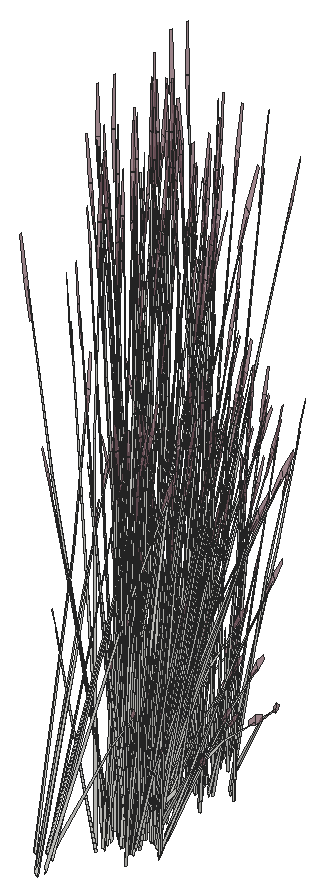
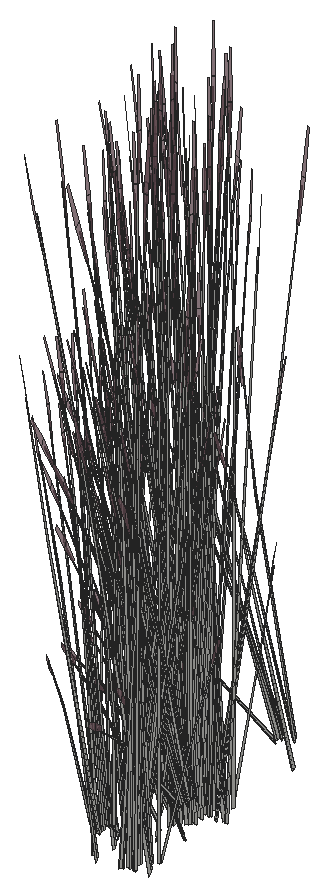
# SketchUp Ruby script. Lengths in inches.
U = 1.inch
M = Sketchup.active_model
def pt(a) = Geom::Point3d.new(a.map { |v| v * U })
def face(e, loops, mat)
  f = e.add_face(loops[0].map { |a| pt(a) })
  loops[1..].each { |l| e.add_face(l.map { |a| pt(a) }).erase! }
  f.material = f.back_material = mat if mat
  f
end
# faces: each face lists its corners as indices into pts; further lists are holes
def faces(e, pts, list, mat = nil) = list.each { |f| face(e, (f[0].is_a?(Array) ? f : [f]).map { |l| l.map { |i| pts[i] } }, mat) }
# xy, xz, yz: faces in a plane at the given z, y or x. An outline is a flat list of corners, or four numbers for a rectangle; further outlines are holes
def ring(l) = l.size == 4 ? [[l[0], l[1]], [l[2], l[1]], [l[2], l[3]], [l[0], l[3]]] : l.each_slice(2).to_a
def flat(e, list, mat, &to3) = list.each { |f| face(e, (f[0].is_a?(Array) ? f : [f]).map { |l| ring(l).map { |u, v| to3.(u, v) } }, mat) }
def xy(e, z, list, mat = nil) = flat(e, list, mat) { |x, y| [x, y, z] }
def xz(e, y, list, mat = nil) = flat(e, list, mat) { |x, z| [x, y, z] }
def yz(e, x, list, mat = nil) = flat(e, list, mat) { |y, z| [x, y, z] }
def lines(e, pts, list) = list.each { |a, b| e.add_line(pt(pts[a]), pt(pts[b])) }
# prism: a flat outline (further loops are holes) pulled along v
def prism(e, loops, v, mat = nil)
  f = face(e, loops, mat); d = Geom::Vector3d.new(v.map { |x| x * U })
  f.pushpull(f.normal.samedirection?(d) ? d.length : -d.length)
end
def box(e, o, s, mat = nil) = prism(e, [[o, [o[0] + s[0], o[1], o[2]], [o[0] + s[0], o[1] + s[1], o[2]], [o[0], o[1] + s[1], o[2]]]], [0, 0, s[2]], mat)
def at(x, y, z, deg = 0) = Geom::Transformation.translation(pt([x, y, z])) * Geom::Transformation.rotation(ORIGIN, Z_AXIS, deg.degrees)
def axes(o, x, y, z) = Geom::Transformation.new([*x, 0, *y, 0, *z, 0, *pt(o).to_a, 1])
def part(name) = M.definitions.add(name)
# library, detail: a bought-in or finely detailed component or shape, given as its bounding box
def library(name, o, s) = part(name).tap { |d| box(d.entities, o, s) }
def detail(e, o, s) = box(e.add_group.entities, o, s)
def put(e, d, t, mat = nil) = e.add_instance(d, t).tap { |i| i.material = mat if mat }
def group(e, t, mat = nil) = e.add_group.tap { |g| g.transformation = t; g.material = mat if mat }.entities
root = M.entities
M.materials.add("LightPink_Translucent").color = [144, 107, 117]
M.materials["LightPink_Translucent"].alpha = 0.75
c1 = part("blade")
p = [[2.15,0.21,22],[0,0.17,0],[0.09,0.45,0],[2.18,0.31,22],[2.29,0.31,22],[0.38,0.45,0],
  [2.48,0.24,33],[2.49,0.24,33],[2.48,0.22,33]]
faces(c1.entities,p,[[0,1,2,3],[4,5,2,3],[6,3,4,7],[8,0,3,6]])
c2 = part("seeds")
p = [[0.3,-0.1,1.38],[-0.01,-0.03,1.59],[-0.01,-0.03,0.03],[0.14,-0.07,-0.07],[0.29,-0.03,3],[0.15,0.01,3.11]]
faces(c2.entities,p,[[0,1,2,3],[1,0,4,5]],"LightPink_Translucent")
c3 = part("blade with seeds")
put(c3.entities,c1,at(0,0,0))
put(c3.entities,c2,axes([2.4,0.25,30.99],[1.5799,-0.05474,1.17369],[-0.12525,1.92788,0.29478],[-0.07173,-0.02425,1.56792]))
put(root,c3,axes([406.99,322.08,-7.34],[0.3661,0.36521,-0.52818],[-0.38674,0.31985,-0.40911],[-0.0557,0.18556,1.01061]))
put(root,c3,axes([406.6,322.63,-9.37],[0.46459,-0.09625,0.0606],[0.10681,0.38778,-0.80367],[-0.02945,0.1963,0.72038]))
put(root,c3,axes([408.08,322.43,-7.64],[0.50273,0.13626,-0.47583],[-0.17232,0.46717,-0.36857],[0.0461,0.18809,0.91046]))
put(root,c3,axes([408.37,321.47,-8.39],[-0.1169,-0.17452,1.59586],[0.54019,-0.14692,0.12904],[0.12209,0.27397,0.68222]))
put(root,c3,axes([407.85,322.72,-7.78],[-0.15418,0.41799,-0.32977],[-0.44981,-0.12192,0.42575],[0.04124,0.16829,0.81462]))
put(root,c3,axes([406.84,330.74,-10.05],[-0.21003,-0.55738,-0.65031],[0.60499,-0.20074,-0.17068],[-0.02321,-0.18874,1.43544]))
put(root,c3,axes([409.65,329.04,-10.61],[-0.07655,-0.04282,1.6421],[-0.19662,-0.47839,-0.25086],[0.13264,-0.12982,0.2797]))
put(root,c3,axes([407.41,321.56,-8.39],[-0.01252,-0.20862,1.59586],[0.54251,0.1384,0.12904],[-0.03356,0.2973,0.68222]))
put(root,c3,axes([408.07,329.15,-7.3],[-0.15418,0.41799,0.32977],[-0.44981,-0.12192,-0.42575],[-0.04124,-0.16829,0.81462]))
put(root,c3,axes([409.22,329.32,-7.59],[0.36417,0.37086,0.447],[-0.38674,0.31985,0.36857],[0.06718,-0.174,0.92496]))
put(root,c3,axes([409.35,329.36,-7.6],[0.42027,0.02533,0.05988],[-0.01152,0.38243,0.47138],[0.04398,-0.14649,0.71878]))
put(root,c3,axes([407.9,322.35,-7.36],[0.24409,0.44196,-0.66157],[-0.50245,0.2463,0.07984],[0.05708,0.21354,0.93586]))
put(root,c3,axes([409.04,329.62,-7.3],[-0.34603,0.28618,0.32977],[-0.32756,-0.32677,-0.42575],[0.04984,-0.16603,0.81462]))
put(root,c3,axes([409.65,330.39,-7.36],[0.26714,-0.42887,-0.66157],[0.46811,0.30479,0.07984],[0.1595,-0.15539,0.93586]))
put(root,c3,axes([406.76,329.14,-9.79],[-0.31974,-0.54466,0],[0.53494,-0.30375,-0.48057],[0.12184,-0.06918,1.52448]))
put(root,c3,axes([409.64,330.1875,-7.64],[-0.13138,-0.49631,-0.47583],[0.49754,-0.08682,-0.36857],[0.14258,-0.13331,0.91046]))
put(root,c3,axes([407.53,323.46,-7.61],[0.06483,0.08753,1.62908],[0.52315,0.03439,-0.25764],[0.05261,0.19303,0.13065]))
put(root,c3,axes([407.46,328.48,-10.02],[-0.35341,0.31182,-0.03625],[-0.32382,-0.34152,-0.16435],[-0.0228,-0.09677,0.54209]))
put(root,c3,axes([409.87,330.54,-7.3125],[-0.47307,-0.29971,-0.11324],[0.27254,-0.43404,-0.62851],[0.13365,-0.15087,0.95501]))
put(root,c3,axes([407.2,329.05,-10.12],[0.47863,-0.27177,-0.46235],[0.28609,0.48733,0],[0.10901,-0.0619,1.46668]))
put(root,c3,axes([410.04,329.99,-9.59],[-0.1827,-0.0161,1.33163],[-0.18717,-0.43188,-0.28638],[0.22444,-0.12218,0.56934]))
put(root,c3,axes([411.04,330.41,-7.62],[-0.0668,-0.00413,1.65179],[-0.27738,-0.44233,-0.15608],[0.11139,-0.14544,0.29231]))
put(root,c3,axes([407.76,330.17,-10.08],[0.34446,-0.40855,-0.58063],[0.42791,0.37046,-0.15239],[0.13803,-0.10191,1.28164]))
put(root,c3,axes([410.25,329.2,-9.42],[-0.17034,0.27669,1.06958],[-0.14642,-0.37174,0.78586],[0.14069,-0.09315,0.23558]))
put(root,c3,axes([410,330.24,-7.78],[0.44516,-0.07768,-0.32977],[0.11755,0.44407,0.42575],[0.12757,-0.11927,0.81462]))
put(root,c3,axes([407.16,330.89,-9.94],[0.24813,-0.48978,-0.41661],[0.51557,0.23571,0.2005],[0,-0.1129,1.33761]))
put(root,c3,axes([407.39,330.64,-9.52],[-0.05959,-0.62022,-0.27094],[0.62068,-0.0375,-0.46562],[0.1093,-0.08261,1.4872]))
put(root,c3,axes([405.85,330.68,-10.11],[0.35699,-0.33913,-0.28847],[0.35699,0.33913,0.28847],[0,-0.10923,1.29413]))
put(root,c3,axes([409.64,330.5,-7.3],[-0.44516,0.07768,0.32977],[-0.11755,-0.44407,-0.42575],[0.12757,-0.11927,0.81462]))
put(root,c3,axes([407.31,329.27,-10.11],[0.47712,0.13449,-0.28847],[-0.12013,0.47362,0.28847],[0.09619,-0.05462,1.29413]))
put(root,c3,axes([410.04,330.43,-7.6],[0.35109,0.22859,0.05988],[-0.2044,0.32553,0.47138],[0.11256,-0.10524,0.71878]))
put(root,c3,axes([409.95,330.34,-7.59],[0.12683,0.50025,0.447],[-0.49754,0.08682,0.36857],[0.14663,-0.11765,0.92496]))
put(root,c3,axes([411.29,330.94,-7.61],[0.07097,-0.08279,1.62908],[-0.09083,-0.50786,-0.25764],[0.17806,-0.09629,0.13065]))
put(root,c3,axes([407.47,331.13,-9.73],[0.57623,0.26344,0.22409],[-0.27732,0.5474,0.46562],[0,-0.12618,1.49497]))
put(root,c3,axes([407.29,330.76,-9.47],[-0.55535,0.03355,0.41661],[-0.05022,-0.55698,-0.2005],[0.09942,-0.05645,1.33761]))
put(root,c3,axes([409.89,331.71,-7.3125],[-0.25732,-0.49218,-0.11324],[0.45669,-0.24187,-0.62851],[0.19245,-0.06494,0.95501]))
put(root,c3,axes([409.87,331.29,-7.64],[0.13855,-0.49442,-0.47583],[0.47502,0.16947,-0.36857],[0.19125,-0.04534,0.91046]))
put(root,c3,axes([409.12,329.28,-9.79],[0.31974,-0.54466,0],[0.53494,0.30375,-0.48057],[0.12184,0.06918,1.52448]))
put(root,c3,axes([407.27,330.96,-9.8],[0.22235,0.6078,0.42607],[-0.63531,0.21135,0.16719],[0.00776,-0.11168,1.47927]))
put(root,c3,axes([410.375,331.43,-10.15],[-0.32938,0.06523,1.31842],[-0.05243,-0.51922,0.07547],[0.2307,-0.07859,0.75023]))
put(root,c3,axes([410.98,330.97,-9.89],[-0.31706,-0.34757,-0.06041],[0.34725,-0.31847,-0.27392],[0.09839,-0.02242,0.90349]))
put(root,c3,axes([407.15,331.44,-9.47],[-0.24813,0.48978,0.41661],[-0.51557,-0.23571,-0.2005],[0,-0.1129,1.33761]))
put(root,c3,axes([408.07,331.01,-9.95],[0,-0.62892,0],[0.63949,0,0],[0,0,1.6711]))
put(root,c3,axes([408.84,329.5625,-9.69],[-0.47863,-0.27177,0.46235],[0.28609,-0.48733,0],[0.10901,0.0619,1.46668]))
put(root,c3,axes([409.78,331.47,-7.36],[0.44939,-0.24006,-0.66157],[0.25044,0.49415,0.07984],[0.21713,-0.05613,0.93586]))
put(root,c3,axes([407.76,330.62,-9.8],[-0.42403,0.49328,0.42607],[-0.50377,-0.43543,0.16719],[0.10223,-0.04923,1.47927]))
put(root,c3,axes([408.23,331.5,-9.86],[-0.47569,-0.46784,-0.05709],[0.47598,-0.46812,0],[-0.01661,-0.01634,1.63492]))
put(root,c3,axes([407.03,329.81,-9.7],[-0.14774,0.54019,0.16428],[-0.54062,-0.15287,0.32672],[0.09339,-0.00263,1.49371]))
put(root,c3,axes([409.71,331.5625,-7.3],[-0.42502,-0.15163,0.32977],[0.12396,-0.44238,-0.42575],[0.17112,-0.04056,0.81462]))
put(root,c3,axes([406.8,330.24,-10.52],[-0.50338,0.21762,1.20058],[-0.16022,-0.62439,0.4665],[0.30911,0.01039,1.36553]))
put(root,c3,axes([408.16,330.41,-9.5625],[0.09866,-0.48509,0.13483],[0.48202,0.0842,-0.38503],[0.08772,0.04981,1.18024]))
put(root,c3,axes([407.32,331.56,-9.8],[0.64638,0.11452,0.42607],[-0.13155,0.64678,0.16719],[-0.09446,-0.06245,1.47927]))
put(root,c3,axes([410.73,331.09,-10.61],[-0.02673,-0.08252,1.6421],[0.18538,-0.48271,-0.25086],[0.187,-0.00694,0.2797]))
put(root,c3,axes([407.95,330.53,-9.47],[-0.30722,-0.45622,0.41661],[0.46535,-0.32126,-0.2005],[0.09942,0.05645,1.33761]))
put(root,c3,axes([406.97,332.59,-9.7],[0.54955,-0.14427,0.16428],[0.1357,0.53689,0.32672],[-0.04901,-0.07823,1.49371]))
put(root,c3,axes([408.11,330.5625,-9.52],[0.51635,-0.36087,-0.27094],[0.34336,0.5099,-0.46562],[0.1274,0.05178,1.4872]))
put(root,c3,axes([410.16,331.51,-7.78],[0.42502,0.15163,-0.32977],[-0.12396,0.44238,0.42575],[0.17112,-0.04056,0.81462]))
put(root,c3,axes([409.41,329.6,-10.12],[0.47863,0.27177,-0.46235],[-0.28609,0.48733,0],[0.10901,0.0619,1.46668]))
put(root,c3,axes([408.5,331.15,-9.95],[0.57217,0,0],[0,0.56272,0],[0,0,1.66132]))
put(root,c3,axes([408.66,329.83,-9.7],[-0.54955,0.14427,0.16428],[-0.1357,-0.53689,0.32672],[0.04901,0.07823,1.49371]))
put(root,c3,axes([409,330.97,-8.39],[-0.21212,0.01231,1.59586],[0.14072,-0.53355,0.12904],[0.3023,0.033,0.68222]))
put(root,c3,axes([409.27,329.81,-10.11],[0.12013,0.47362,-0.28847],[-0.47712,0.13449,0.28847],[0.09619,0.05462,1.29413]))
put(root,c3,axes([410.1,331.7,-7.6],[0.18783,0.37061,0.05988],[-0.34252,0.1814,0.47138],[0.15099,-0.03579,0.71878]))
put(root,c3,axes([408.31,330.87,-9.78],[-0.64638,-0.11452,0.45814],[0.13155,-0.64678,0.17978],[0.09446,0.06245,1.59061]))
put(root,c3,axes([410.06,331.57,-7.59],[-0.14449,0.4956,0.447],[-0.47502,-0.16947,0.36857],[0.1868,-0.02978,0.92496]))
put(root,c3,axes([407.8,332.46,-9.95],[-0.16686,-0.46861,0],[0.47648,-0.16411,0],[0,0,1.4375]))
put(root,c3,axes([408.42,332.4,-9.97],[0.53691,-0.18442,-0.17877],[0.18866,0.53125,0.00007],[0.05927,-0.02038,1.61933]))
put(root,c3,axes([408.61,332.62,-9.7],[0.14774,-0.54019,0.16428],[0.54062,0.15287,0.32672],[-0.09339,0.00263,1.49371]))
put(root,c3,axes([408.49,331.4,-9.9375],[0.35699,0.35109,0],[-0.35699,0.35109,0],[0,0,1.57621]))
put(root,c3,axes([409.45,331.24,-9.7],[-0.40181,-0.39593,0.16428],[0.40492,-0.38402,0.32672],[-0.04438,0.08086,1.49371]))
put(root,c3,axes([408.71,330.64,-10.08],[0.53199,0.08911,-0.58063],[-0.11226,0.54969,-0.15239],[0.15876,0.06661,1.28164]))
put(root,c3,axes([411.0625,331.6,-9.42],[-0.31598,0.08973,1.06958],[0.14873,-0.37085,0.78586],[0.16763,0.02538,0.23558]))
put(root,c3,axes([407.68,332.68,-9.95],[-0.51557,-0.24403,0],[0.24813,-0.50705,0],[0,0,1.51513]))
put(root,c3,axes([408.48,330.98,-9.47],[0.24813,-0.48978,0.41661],[0.51557,0.23571,-0.2005],[0,0.1129,1.33761]))
put(root,c3,axes([410.91,333.17,-7.62],[-0.04624,-0.04758,1.65179],[0.10116,-0.51007,-0.15608],[0.18215,-0.03259,0.29231]))
put(root,c3,axes([408.39,331.27,-9.87],[0,0.62861,-0.05249],[-0.63949,0,0],[0,0.01975,1.67027]))
put(root,c3,axes([408.43,330.82,-9.94],[0.30722,0.45622,-0.41661],[-0.46535,0.32126,0.2005],[0.09942,0.05645,1.33761]))
put(root,c3,axes([410.51,332.75,-8.34],[-0.09788,-0.45691,-0.03251],[0.46264,-0.10504,-0.14742],[0.09661,0.02897,0.48626]))
put(root,c3,axes([409.3125,332.73,-7.3125],[0.02738,-0.55277,-0.11324],[0.51847,0.01511,-0.62851],[0.19968,0.0384,0.95501]))
put(root,c3,axes([409.78,331.26,-9.69],[0,-0.54355,0.46235],[0.57217,0,0],[0,0.1238,1.46668]))
put(root,c3,axes([408.35,331.66,-9.47],[0.55535,-0.03355,0.41661],[0.05022,0.55698,-0.2005],[-0.09942,0.05645,1.33761]))
put(root,c3,axes([408.7,331.1,-9.5625],[0.47648,-0.15851,0.13483],[0.16686,0.45265,-0.38503],[0,0.09962,1.18024]))
put(root,c3,axes([409.23,332.52,-7.3],[-0.29098,-0.34031,0.32977],[0.33226,-0.32215,-0.42575],[0.16881,0.04902,0.81462]))
put(root,c3,axes([410.47,332.2,-9.59],[-0.12317,-0.13368,1.33163],[0.16025,-0.44223,-0.28638],[0.24919,0.05991,0.56934]))
put(root,c3,axes([408.27,332.6875,-9.95],[0.51557,0.24403,0],[-0.24813,0.50705,0],[0,0,1.62917]))
put(root,c3,axes([409.76,332.4,-7.61],[0.10971,-0.00919,1.62908],[0.30091,-0.42228,-0.25764],[0.19514,0.05574,0.13065]))
put(root,c3,axes([408.36,331.9,-9.5625],[0.37783,0.32657,0.13483],[-0.31516,0.36844,-0.38503],[-0.08772,0.04981,1.18024]))
put(root,c3,axes([407.88,337.63,-9.59],[-0.14537,0.11002,1.33163],[-0.43536,-0.19256,-0.28638],[0.0807,-0.23948,0.56934]))
put(root,c3,axes([409.34,332.47,-7.36],[0.51122,0.01309,-0.66157],[-0.03434,0.5511,0.07984],[0.21658,0.05816,0.93586]))
put(root,c3,axes([406.79,337.03,-10.61],[-0.08578,0.01958,1.6421],[-0.47437,-0.22044,-0.25086],[0.00796,-0.18387,0.2797]))
put(root,c3,axes([408.76,332.91,-9.69],[0.47863,-0.27177,0.46235],[0.28609,0.48733,0],[-0.10901,0.0619,1.46668]))
put(root,c3,axes([408.08,332.48,-9.87],[0.22235,0.62444,-0.05599],[-0.63531,0.21881,0],[0.00776,0.02181,1.60327]))
put(root,c3,axes([408.23,338.45,-7.36],[0.01331,-0.50278,-0.66157],[0.56035,0.03377,0.07984],[0.05914,-0.213,0.93586]))
put(root,c3,axes([410.17,331.35,-9.79],[0.63949,0,0],[0,0.60749,-0.48057],[0,0.13836,1.52448]))
put(root,c3,axes([409.01,337.66,-7.61],[-0.00494,-0.10818,1.62908],[-0.41695,-0.31265,-0.25764],[0.06446,-0.18952,0.13065]))
put(root,c3,axes([407.26,337.64,-7.78],[0.15418,-0.41799,-0.32977],[0.44981,0.12192,0.42575],[-0.04124,-0.16829,0.81462]))
put(root,c3,axes([407.6,338.19,-8.39],[-0.09522,0.18683,1.59586],[-0.39947,-0.38663,0.12904],[0.18021,-0.24097,0.68222]))
put(root,c3,axes([408.9,337.27,-7.62],[-0.05194,0.04152,1.65179],[-0.50886,-0.14007,-0.15608],[-0.01842,-0.18118,0.29231]))
put(root,c3,axes([409.92,331.66,-9.95],[-0.63917,-0.00435,-0.04634],[0,-0.60749,0.46507],[-0.02009,0.13829,1.47457]))
put(root,c3,axes([408.53,331.13,-9.52],[0.57594,0.25935,-0.27094],[-0.27732,0.5474,-0.46562],[0.0181,0.1344,1.4872]))
put(root,c3,axes([409.65,332.7,-7.78],[0.29098,0.34031,-0.32977],[-0.33226,0.32215,0.42575],[0.16881,0.04902,0.81462]))
put(root,c3,axes([409.78,331.75,-10.11],[-0.35699,0.33913,-0.28847],[-0.35699,-0.33913,0.28847],[0,0.10923,1.29413]))
put(root,c3,axes([408.25,331.78,-9.52],[0.05959,0.62022,-0.27094],[-0.62068,0.0375,-0.46562],[-0.1093,0.08261,1.4872]))
put(root,c3,axes([409.5,332.83,-7.6],[-0.02575,0.41332,0.05988],[-0.38885,-0.01133,0.47138],[0.14895,0.04325,0.71878]))
put(root,c3,axes([407.34,336.76,-9.42],[0.06561,0.31695,1.06958],[-0.36394,-0.17555,0.78586],[0.03916,-0.16229,0.23558]))
put(root,c3,axes([408.47,331.54,-9.94],[-0.24813,0.48978,-0.41661],[-0.51557,-0.23571,0.2005],[0,0.1129,1.33761]))
put(root,c3,axes([408.12,338.28,-7.64],[-0.3661,-0.36521,-0.47583],[0.38674,-0.31985,-0.36857],[0.0557,-0.18556,0.91046]))
put(root,c3,axes([409.53,332.69,-7.59],[-0.37709,0.35815,0.447],[-0.32522,-0.38035,0.36857],[0.17692,0.06607,0.92496]))
put(root,c3,axes([407.32,337.74,-7.59],[0.50393,0.1421,0.447],[-0.17232,0.46717,0.36857],[-0.03028,-0.18372,0.92496]))
put(root,c3,axes([408.33,333.11,-7.3],[-0.07899,-0.43781,0.32977],[0.45153,-0.11561,-0.42575],[0.12128,0.12546,0.81462]))
put(root,c3,axes([408.49,332.95,-9.83],[0.64025,0.17667,0.2864],[-0.16018,0.63149,-0.33981],[-0.10597,0.07904,1.53541]))
put(root,c3,axes([408.5,338.47,-7.3125],[-0.56206,-0.02693,-0.11324],[0.01536,-0.50991,-0.62851],[0.03904,-0.19638,0.95501]))
put(root,c3,axes([410.03,331.76,-10.12],[0,0.54355,-0.46235],[-0.57217,0,0],[0,0.1238,1.46668]))
put(root,c3,axes([408.46,338.14,-7.78],[0.34603,-0.28618,-0.32977],[0.32756,0.32677,0.42575],[0.04984,-0.16603,0.81462]))
put(root,c3,axes([407.45,337.7,-7.6],[0.37684,-0.18473,0.05988],[0.18445,0.33686,0.47138],[-0.03639,-0.14849,0.71878]))
put(root,c3,axes([408.6,331.82,-8.39],[-0.18996,-0.09365,1.59586],[0.39312,-0.39287,0.12904],[0.24502,0.17723,0.68222]))
put(root,c3,axes([408.64,330.59,-7.83],[-0.44191,-0.28242,1.28769],[0.46662,-0.43971,0.5556],[0.14258,0.26499,1.24467]))
put(root,c3,axes([409.3,332.89,-9.42],[-0.28795,-0.15629,1.06958],[0.37181,-0.1588,0.78586],[0.10029,0.13452,0.23558]))
put(root,c3,axes([408.29,333.34,-7.3125],[0.30474,-0.46525,-0.11324],[0.44133,0.26804,-0.62851],[0.15341,0.13145,0.95501]))
put(root,c3,axes([408.875,333.29,-9.79],[0.31974,0.54466,0],[-0.53494,0.30375,-0.48057],[-0.12184,0.06918,1.52448]))
put(root,c3,axes([407.89,333.72,-7.62],[0.00151,-0.06581,1.65179],[0.43826,-0.29033,-0.15608],[0.15223,0.10363,0.29231]))
put(root,c3,axes([408.89,337.97,-10.61],[-0.07655,-0.04282,1.6421],[-0.19662,-0.47839,-0.25086],[0.13264,-0.12982,0.2797]))
put(root,c3,axes([409.38,333.47,-10.61],[0.03726,-0.07847,1.6421],[0.46909,-0.23111,-0.25086],[0.14221,0.11962,0.2797]))
put(root,c3,axes([408.76,331.6875,-10.05],[0.18752,0.49766,-0.6445],[-0.54017,0.17923,-0.16915],[0.02073,0.16852,1.42262]))
put(root,c3,axes([408.65,333.11,-7.64],[0.50465,-0.12921,-0.47583],[0.08828,0.48932,-0.36857],[0.13555,0.14022,0.91046]))
put(root,c3,axes([407.3125,338.08,-7.3],[-0.15418,0.41799,0.32977],[-0.44981,-0.12192,-0.42575],[-0.04124,-0.16829,0.81462]))
put(root,c3,axes([407.25,333.18,-7.3],[0.15418,-0.41799,0.32977],[0.44981,0.12192,-0.42575],[0.04124,0.16829,0.81462]))
put(root,c3,axes([408.46,338.26,-7.59],[0.36417,0.37086,0.447],[-0.38674,0.31985,0.36857],[0.06718,-0.174,0.92496]))
put(root,c3,axes([408.59,338.29,-7.6],[0.42027,0.02533,0.05988],[-0.01152,0.38243,0.47138],[0.04398,-0.14649,0.71878]))
put(root,c3,axes([409.35,333.6,-9.52],[-0.32795,-0.01705,0.97832],[0.21658,-0.36206,0.54015],[0.12956,0.12863,0.76741]))
put(root,c3,axes([408.28,338.55,-7.3],[-0.34603,0.28618,0.32977],[-0.32756,-0.32677,-0.42575],[0.04984,-0.16603,0.81462]))
put(root,c3,axes([408.89,339.32,-7.36],[0.26714,-0.42887,-0.66157],[0.46811,0.30479,0.07984],[0.1595,-0.15539,0.93586]))
put(root,c3,axes([408.4,333.51,-7.6],[-0.23243,0.34529,0.05988],[-0.331,-0.20103,0.47138],[0.10701,0.1107,0.71878]))
put(root,c3,axes([406,338.07,-9.79],[-0.31974,-0.54466,0],[0.53494,-0.30375,-0.48057],[0.12184,-0.06918,1.52448]))
put(root,c3,axes([408.88,339.12,-7.64],[-0.13138,-0.49631,-0.47583],[0.49754,-0.08682,-0.36857],[0.14258,-0.13331,0.91046]))
put(root,c3,axes([407.86,334.67,-6.74],[0.35341,-0.31182,-0.06041],[0.32382,0.34152,-0.27392],[0.0228,0.09677,0.90349]))
put(root,c3,axes([408.5,333.41,-7.59],[-0.50866,0.12474,0.447],[-0.08828,-0.48932,0.36857],[0.11963,0.14421,0.92496]))
put(root,c3,axes([409.11,339.48,-7.3125],[-0.47307,-0.29971,-0.11324],[0.27254,-0.43404,-0.62851],[0.13365,-0.15087,0.95501]))
put(root,c3,axes([408.28,332.72,-9.59],[0.00902,-0.18018,1.33163],[0.43127,-0.20126,-0.28638],[0.13313,0.21566,0.56934]))
put(root,c3,axes([407.11,333.56,-7.6],[-0.37684,0.18473,0.05988],[-0.18445,-0.33686,0.47138],[0.03639,0.14849,0.71878]))
put(root,c3,axes([407.1,333.35,-7.3125],[0.50045,-0.25306,-0.11324],[0.24593,0.44915,-0.62851],[0.06603,0.18927,0.95501]))
put(root,c3,axes([407.25,333.52,-7.28],[-0.50393,-0.1421,0.49617],[0.17232,-0.46717,0.40911],[0.03028,0.18372,1.0267]))
put(root,c3,axes([406.4375,337.99,-10.12],[0.47863,-0.27177,-0.46235],[0.28609,0.48733,0],[0.10901,-0.0619,1.46668]))
put(root,c3,axes([409.28,338.93,-9.59],[-0.1827,-0.0161,1.33163],[-0.18717,-0.43188,-0.28638],[0.22444,-0.12218,0.56934]))
put(root,c3,axes([410.28,339.35,-7.62],[-0.0668,-0.00413,1.65179],[-0.27738,-0.44233,-0.15608],[0.11139,-0.14544,0.29231]))
put(root,c3,axes([407.01,339.1,-10.08],[0.34446,-0.40855,-0.58063],[0.42791,0.37046,-0.15239],[0.13803,-0.10191,1.28164]))
put(root,c3,axes([407.19,333.45,-10.61],[0.08277,-0.02958,1.6421],[0.49786,0.16279,-0.25086],[0.01456,0.18348,0.2797]))
put(root,c3,axes([409.49,338.13,-9.42],[-0.17034,0.27669,1.06958],[-0.14642,-0.37174,0.78586],[0.14069,-0.09315,0.23558]))
put(root,c3,axes([409.25,339.17,-7.78],[0.44516,-0.07768,-0.32977],[0.11755,0.44407,0.42575],[0.12757,-0.11927,0.81462]))
put(root,c3,axes([407.53,333.33,-7.64],[0.50273,0.13626,-0.47583],[-0.17232,0.46717,-0.36857],[0.0461,0.18809,0.91046]))
put(root,c3,axes([407.82,332.37,-8.39],[-0.1169,-0.17452,1.59586],[0.54019,-0.14692,0.12904],[0.12209,0.27397,0.68222]))
put(root,c3,axes([406.41,339.82,-9.94],[0.24813,-0.48978,-0.41661],[0.51557,0.23571,0.2005],[0,-0.1129,1.33761]))
put(root,c3,axes([406.63,339.58,-9.52],[-0.05959,-0.62022,-0.27094],[0.62068,-0.0375,-0.46562],[0.1093,-0.08261,1.4872]))
put(root,c3,axes([407.3,333.62,-7.78],[-0.15418,0.41799,-0.32977],[-0.44981,-0.12192,0.42575],[0.04124,0.16829,0.81462]))
put(root,c3,axes([408.88,339.44,-7.3],[-0.44516,0.07768,0.32977],[-0.11755,-0.44407,-0.42575],[0.12757,-0.11927,0.81462]))
put(root,c3,axes([406.55,338.2,-10.11],[0.47712,0.13449,-0.28847],[-0.12013,0.47362,0.28847],[0.09619,-0.05462,1.29413]))
put(root,c3,axes([406.86,332.45,-8.39],[-0.01252,-0.20862,1.59586],[0.54251,0.1384,0.12904],[-0.03356,0.2973,0.68222]))
put(root,c3,axes([407.35,333.24,-7.36],[0.24409,0.44196,-0.66157],[-0.50245,0.2463,0.07984],[0.05708,0.21354,0.93586]))
put(root,c3,axes([409.29,339.36,-7.6],[0.35109,0.22859,0.05988],[-0.2044,0.32553,0.47138],[0.11256,-0.10524,0.71878]))
put(root,c3,axes([409.1875,339.27,-7.59],[0.12683,0.50025,0.447],[-0.49754,0.08682,0.36857],[0.14663,-0.11765,0.92496]))
put(root,c3,axes([410.53,339.875,-7.61],[0.07097,-0.08279,1.62908],[-0.09083,-0.50786,-0.25764],[0.17806,-0.09629,0.13065]))
put(root,c3,axes([406.98,334.36,-7.61],[0.06483,0.08753,1.62908],[0.52315,0.03439,-0.25764],[0.05261,0.19303,0.13065]))
put(root,c3,axes([406.71,340.0625,-9.73],[0.57623,0.26344,0.22409],[-0.27732,0.5474,0.46562],[0,-0.12618,1.49497]))
put(root,c3,axes([406.53,339.7,-9.47],[-0.55535,0.03355,0.41661],[-0.05022,-0.55698,-0.2005],[0.09942,-0.05645,1.33761]))
put(root,c3,axes([409.13,340.65,-7.3125],[-0.25732,-0.49218,-0.11324],[0.45669,-0.24187,-0.62851],[0.19245,-0.06494,0.95501]))
put(root,c3,axes([409.11,340.22,-7.64],[0.13855,-0.49442,-0.47583],[0.47502,0.16947,-0.36857],[0.19125,-0.04534,0.91046]))
put(root,c3,axes([408.36,338.21,-9.79],[0.31974,-0.54466,0],[0.53494,0.30375,-0.48057],[0.12184,0.06918,1.52448]))
put(root,c3,axes([406.51,339.9,-9.8],[0.22235,0.6078,0.42607],[-0.63531,0.21135,0.16719],[0.00776,-0.11168,1.47927]))
put(root,c3,axes([409.62,340.36,-10.15],[-0.32938,0.06523,1.31842],[-0.05243,-0.51922,0.07547],[0.2307,-0.07859,0.75023]))
put(root,c3,axes([410.22,339.9,-9.89],[-0.31706,-0.34757,-0.06041],[0.34725,-0.31847,-0.27392],[0.09839,-0.02242,0.90349]))
put(root,c3,axes([407.31,339.95,-9.95],[0,-0.62892,0],[0.63949,0,0],[0,0,1.6711]))
put(root,c3,axes([408.08,338.49,-9.69],[-0.47863,-0.27177,0.46235],[0.28609,-0.48733,0],[0.10901,0.0619,1.46668]))
put(root,c3,axes([409.02,340.4,-7.36],[0.44939,-0.24006,-0.66157],[0.25044,0.49415,0.07984],[0.21713,-0.05613,0.93586]))
put(root,c3,axes([407,339.55,-9.8],[-0.42403,0.49328,0.42607],[-0.50377,-0.43543,0.16719],[0.10223,-0.04923,1.47927]))
put(root,c3,axes([407.47,340.43,-9.86],[-0.47569,-0.46784,-0.05709],[0.47598,-0.46812,0],[-0.01661,-0.01634,1.63492]))
put(root,c3,axes([406.27,338.74,-9.7],[-0.14774,0.54019,0.16428],[-0.54062,-0.15287,0.32672],[0.09339,-0.00263,1.49371]))
put(root,c3,axes([408.95,340.5,-7.3],[-0.42502,-0.15163,0.32977],[0.12396,-0.44238,-0.42575],[0.17112,-0.04056,0.81462]))
put(root,c3,axes([406.04,339.18,-10.52],[-0.50338,0.21762,1.20058],[-0.16022,-0.62439,0.4665],[0.30911,0.01039,1.36553]))
put(root,c3,axes([407.4,339.34,-9.5625],[0.09866,-0.48509,0.13483],[0.48202,0.0842,-0.38503],[0.08772,0.04981,1.18024]))
